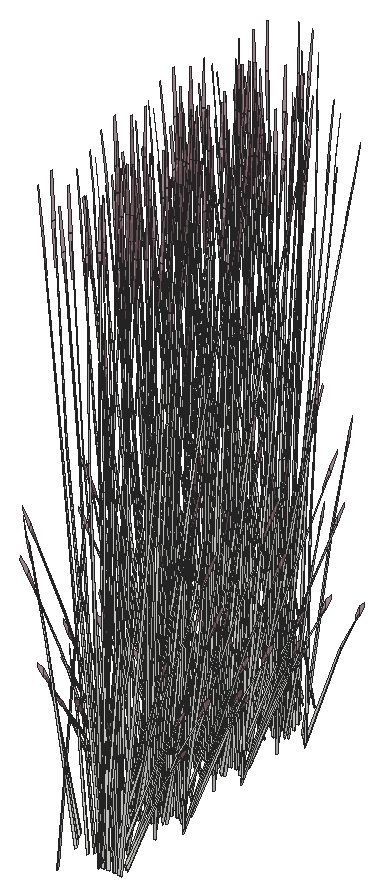
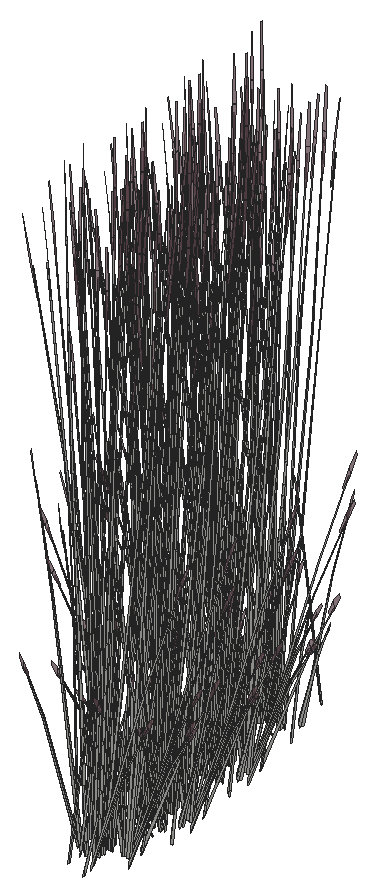
# SketchUp Ruby script. Lengths in inches.
U = 1.inch
M = Sketchup.active_model
def pt(a) = Geom::Point3d.new(a.map { |v| v * U })
def face(e, loops, mat)
  f = e.add_face(loops[0].map { |a| pt(a) })
  loops[1..].each { |l| e.add_face(l.map { |a| pt(a) }).erase! }
  f.material = f.back_material = mat if mat
  f
end
# faces: each face lists its corners as indices into pts; further lists are holes
def faces(e, pts, list, mat = nil) = list.each { |f| face(e, (f[0].is_a?(Array) ? f : [f]).map { |l| l.map { |i| pts[i] } }, mat) }
# xy, xz, yz: faces in a plane at the given z, y or x. An outline is a flat list of corners, or four numbers for a rectangle; further outlines are holes
def ring(l) = l.size == 4 ? [[l[0], l[1]], [l[2], l[1]], [l[2], l[3]], [l[0], l[3]]] : l.each_slice(2).to_a
def flat(e, list, mat, &to3) = list.each { |f| face(e, (f[0].is_a?(Array) ? f : [f]).map { |l| ring(l).map { |u, v| to3.(u, v) } }, mat) }
def xy(e, z, list, mat = nil) = flat(e, list, mat) { |x, y| [x, y, z] }
def xz(e, y, list, mat = nil) = flat(e, list, mat) { |x, z| [x, y, z] }
def yz(e, x, list, mat = nil) = flat(e, list, mat) { |y, z| [x, y, z] }
def lines(e, pts, list) = list.each { |a, b| e.add_line(pt(pts[a]), pt(pts[b])) }
# prism: a flat outline (further loops are holes) pulled along v
def prism(e, loops, v, mat = nil)
  f = face(e, loops, mat); d = Geom::Vector3d.new(v.map { |x| x * U })
  f.pushpull(f.normal.samedirection?(d) ? d.length : -d.length)
end
def box(e, o, s, mat = nil) = prism(e, [[o, [o[0] + s[0], o[1], o[2]], [o[0] + s[0], o[1] + s[1], o[2]], [o[0], o[1] + s[1], o[2]]]], [0, 0, s[2]], mat)
def at(x, y, z, deg = 0) = Geom::Transformation.translation(pt([x, y, z])) * Geom::Transformation.rotation(ORIGIN, Z_AXIS, deg.degrees)
def axes(o, x, y, z) = Geom::Transformation.new([*x, 0, *y, 0, *z, 0, *pt(o).to_a, 1])
def part(name) = M.definitions.add(name)
# library, detail: a bought-in or finely detailed component or shape, given as its bounding box
def library(name, o, s) = part(name).tap { |d| box(d.entities, o, s) }
def detail(e, o, s) = box(e.add_group.entities, o, s)
def put(e, d, t, mat = nil) = e.add_instance(d, t).tap { |i| i.material = mat if mat }
def group(e, t, mat = nil) = e.add_group.tap { |g| g.transformation = t; g.material = mat if mat }.entities
root = M.entities
M.materials.add("LightPink_Translucent").color = [144, 107, 117]
M.materials["LightPink_Translucent"].alpha = 0.75
c1 = part("blade")
p = [[2.15,0.21,22],[0,0.17,0],[0.09,0.45,0],[2.18,0.31,22],[2.29,0.31,22],[0.38,0.45,0],
  [2.48,0.24,33],[2.49,0.24,33],[2.48,0.22,33]]
faces(c1.entities,p,[[0,1,2,3],[4,5,2,3],[6,3,4,7],[8,0,3,6]])
c2 = part("seeds")
p = [[0.3,-0.1,1.38],[-0.01,-0.03,1.59],[-0.01,-0.03,0.03],[0.14,-0.07,-0.07],[0.29,-0.03,3],[0.15,0.01,3.11]]
faces(c2.entities,p,[[0,1,2,3],[1,0,4,5]],"LightPink_Translucent")
c3 = part("blade with seeds")
put(c3.entities,c1,at(0,0,0))
put(c3.entities,c2,axes([2.4,0.25,30.99],[1.5799,-0.05474,1.17369],[-0.12525,1.92788,0.29478],[-0.07173,-0.02425,1.56792]))
put(root,c3,axes([430.54,388.57,152.09],[-0.32198,-0.34356,0.14904],[0.32447,-0.33323,0.29641],[-0.03556,0.07016,1.35512]))
put(root,c3,axes([431.83,388.88,152.34],[-0.2532,0.07787,0.97034],[0.11918,-0.32181,0.71294],[0.13432,0.02202,0.21373]))
put(root,c3,axes([429.12,389.8125,151.86],[-0.41314,-0.21175,0],[0.19883,-0.43999,0],[0,0,1.37455]))
put(root,c3,axes([429.46,389.25,152.08],[-0.40016,-0.37963,-0.21282],[0.33672,-0.42629,0.46574],[-0.10776,0.04441,1.42109]))
put(root,c3,axes([428.41,389.98,152.09],[0.38354,0.23583,0.41945],[-0.22925,0.42288,0],[-0.08735,-0.05371,1.33059]))
put(root,c3,axes([429.76,388.35,152.3],[0.19883,-0.425,0.37796],[0.41314,0.20454,-0.1819],[0,0.09797,1.2135]))
put(root,c3,axes([429.68,388.59,151.9375],[0,0.54548,-0.04762],[-0.51243,0,0],[0,0.01714,1.5153]))
put(root,c3,axes([428.1875,390.22,152],[-0.25622,0.47263,0],[-0.42866,-0.26357,-0.43598],[-0.09763,-0.06003,1.38303]))
put(root,c3,axes([427.72,386.34,152.1875],[0.12932,-0.07441,1.20808],[0.31929,0.22435,-0.25981],[-0.09503,0.19413,0.51652]))
put(root,c3,axes([430.8,388.58,152.09],[0,-0.47166,0.41945],[0.45849,0,0],[0,0.10742,1.33059]))
put(root,c3,axes([429.66,388.93,152.3],[0.44501,-0.02912,0.37796],[0.04024,0.48332,-0.1819],[-0.07967,0.04899,1.2135]))
put(root,c3,axes([429.93,388.44,152.21],[0.38182,-0.13755,0.12232],[0.13371,0.39278,-0.3493],[0,0.08644,1.07074]))
put(root,c3,axes([431.35,389.4,152.1875],[-0.0987,-0.116,1.20808],[0.12841,-0.38374,-0.25981],[0.19968,0.05198,0.51652]))
put(root,c3,axes([429.59,389.82,151.86],[0.41314,0.21175,0],[-0.19883,0.43999,0],[0,0,1.47801]))
put(root,c3,axes([429.75,390.29,151.85],[-0.25302,-0.47428,-0.04344],[0.42866,-0.26357,0.43598],[-0.10563,0.04516,1.38235]))
put(root,c3,axes([429.66,389.14,152.21],[0.30276,0.28338,0.12232],[-0.25254,0.31972,-0.3493],[-0.07029,0.04322,1.07074]))
put(root,c3,axes([429.99,390.02,152.09],[0.38354,-0.23583,0.41945],[0.22925,0.42288,0],[-0.08735,0.05371,1.33059]))
put(root,c3,axes([429.44,389.64,151.9375],[0.17817,0.54185,-0.05079],[-0.50909,0.18987,0],[0.00622,0.01892,1.45452]))
put(root,c3,axes([426.88,389.4,152.1875],[0.14242,0.03872,1.20808],[0.09179,0.39548,-0.25981],[-0.19345,0.07403,0.51652]))
put(root,c3,axes([431.12,388.66,152.01],[0.51243,0,0],[0,0.52715,-0.43598],[0,0.12006,1.38303]))
put(root,c3,axes([430.91,388.93,151.86],[-0.51218,-0.00377,-0.04204],[0,-0.52715,0.42192],[-0.0161,0.12,1.33776]))
put(root,c3,axes([429.8,388.47,152.25],[0.46151,0.22505,-0.2458],[-0.22222,0.475,-0.42242],[0.0145,0.11662,1.34921]))
put(root,c3,axes([426.58,390.22,152.34],[0.17079,-0.21377,0.97034],[0.06739,0.33841,0.71294],[-0.12342,0.0606,0.21373]))
put(root,c3,axes([429.57,389.04,152.25],[0.04775,0.53819,-0.2458],[-0.49736,0.03254,-0.42242],[-0.08758,0.07169,1.34921]))
put(root,c3,axes([428.53,394.79,152.1875],[-0.11649,0.09547,1.20808],[-0.34886,-0.1671,-0.25981],[0.06467,-0.20781,0.51652]))
put(root,c3,axes([426.72,394.61,152.1875],[-0.02482,0.15429,1.20808],[-0.36278,0.12916,-0.25981],[-0.0848,-0.19943,0.51652]))
put(root,c3,axes([427.66,394.27,151.26],[-0.06874,0.01699,1.48974],[-0.38012,-0.19128,-0.22758],[0.00638,-0.15955,0.25375]))
put(root,c3,axes([429.76,390.05,151.97],[0.51304,0.1533,0.25983],[-0.12835,0.54797,-0.30828],[-0.08491,0.06858,1.39295]))
put(root,c3,axes([428.1,394.03,152.34],[0.05257,0.27504,0.97034],[-0.29163,-0.15233,0.71294],[0.03138,-0.14083,0.21373]))
put(root,c3,axes([430.42,390,152.34],[-0.23074,-0.13562,0.97034],[0.29794,-0.1378,0.71294],[0.08036,0.11673,0.21373]))
put(root,c3,axes([430.08,390.34,152],[0.25622,0.47263,0],[-0.42866,0.26357,-0.43598],[-0.09763,0.06003,1.38303]))
put(root,c3,axes([430.48,390.5,151.26],[0.02986,-0.06809,1.48974],[0.37589,-0.20055,-0.22758],[0.11396,0.1038,0.25375]))
put(root,c3,axes([429.86,388.47,152.4],[-0.01119,-0.44408,1.19347],[0.50665,0.11511,0.50532],[-0.11983,0.243,1.12654]))
put(root,c3,axes([427.03,390.44,151.26],[0.05497,0.04712,1.48974],[0.09321,0.43661,-0.22758],[-0.12183,0.0931,0.25375]))
put(root,c3,axes([426.6,394.36,152.34],[0.21377,0.16416,0.97034],[-0.31132,0.09868,0.71294],[-0.06661,-0.12616,0.21373]))
put(root,c3,axes([430.46,390.62,152.25],[-0.26279,-0.01479,0.88755],[0.17355,-0.31417,0.49003],[0.10382,0.11162,0.6962]))
put(root,c3,axes([426.43,394.85,151.26],[-0.0397,0.06213,1.48974],[-0.40116,0.13396,-0.22758],[-0.09691,-0.12186,0.25375]))
put(root,c3,axes([429.34,395.08,151.26],[-0.06134,-0.03716,1.48974],[-0.15755,-0.41512,-0.22758],[0.10629,-0.11265,0.25375]))
put(root,c3,axes([429.6,389.85,152.1875],[0.00723,-0.15635,1.20808],[0.34559,-0.17464,-0.25981],[0.10668,0.18713,0.51652]))
put(root,c3,axes([428.03,391.16,152.34],[-0.01061,-0.28045,0.97034],[0.26501,0.20003,0.71294],[-0.05212,0.13367,0.21373]))
put(root,c3,axes([427.03,395.17,152],[-0.25622,-0.47263,0],[0.42866,-0.26357,-0.43598],[0.09763,-0.06003,1.38303]))
put(root,c3,axes([428.73,390.49,151.26],[0.06632,-0.02567,1.48974],[0.39894,0.14126,-0.22758],[0.01167,0.15921,0.25375]))
put(root,c3,axes([427.59,394.6,151.8],[-0.28319,0.27058,-0.03288],[-0.25948,-0.29635,-0.1491],[-0.01827,-0.08397,0.4918]))
put(root,c3,axes([427.8125,390.55,152.38],[0.37228,-0.08352,0.05498],[0.08559,0.3365,-0.7291],[-0.0236,0.17034,0.65354]))
put(root,c3,axes([429.65,395.91,152.1875],[-0.1464,-0.01397,1.20808],[-0.14998,-0.37477,-0.25981],[0.17985,-0.10602,0.51652]))
put(root,c3,axes([429.82,395.22,152.34],[-0.1365,0.2401,0.97034],[-0.11733,-0.32258,0.71294],[0.11274,-0.08083,0.21373]))
put(root,c3,axes([427.72,390.91,152.1875],[0.12932,-0.07441,1.20808],[0.31929,0.22435,-0.25981],[-0.09503,0.19413,0.51652]))
put(root,c3,axes([427.53,396.47,152.25],[-0.04775,-0.53819,-0.2458],[0.49736,-0.03254,-0.42242],[0.08758,-0.07169,1.34921]))
put(root,c3,axes([426.18,395.09,151.8],[-0.11822,0.38513,-0.03288],[-0.36385,-0.11847,-0.1491],[-0.05524,-0.06299,0.4918]))
put(root,c3,axes([427.3,397.04,152.25],[-0.46151,-0.22505,-0.2458],[0.22222,-0.475,-0.42242],[-0.0145,-0.11662,1.34921]))
put(root,c3,axes([425.99,396.85,152],[-0.51243,0,0],[0,-0.52715,-0.43598],[0,-0.12006,1.38303]))
put(root,c3,axes([426.07,395.91,152.1875],[0.08001,0.13132,1.20808],[-0.18437,0.35694,-0.25981],[-0.18931,-0.08532,0.51652]))
put(root,c3,axes([426.38,396.71,151.97],[-0.38118,0.39654,0.25983],[-0.38142,-0.39237,-0.30828],[-0.01331,-0.11261,1.39295]))
put(root,c3,axes([427.59,396.9,152.06],[0.46174,0.2286,0.2033],[-0.22222,0.475,0.42242],[0,-0.1095,1.35626]))
put(root,c3,axes([427.41,397.54,152.06],[0.10862,-0.55889,-0.19793],[0.515,0.09742,0.43313],[-0.08999,-0.07718,1.32161]))
put(root,c3,axes([425.6,396.3,152.34],[0.26163,-0.03375,0.97034],[-0.16596,0.29737,0.71294],[-0.12929,-0.04461,0.21373]))
put(root,c3,axes([427.45,396.58,152.3],[-0.44501,0.02912,0.37796],[-0.04024,-0.48332,-0.1819],[0.07967,-0.04899,1.2135]))
put(root,c3,axes([426.3,396.93,152.09],[0,0.47166,0.41945],[-0.45849,0,0],[0,-0.10742,1.33059]))
put(root,c3,axes([428.91,395.29,152.01],[0.25622,-0.47263,0],[0.42866,0.26357,-0.43598],[0.09763,0.06003,1.38303]))
put(root,c3,axes([427.43,396.75,151.99],[0.17817,0.52741,0.38653],[-0.50909,0.1834,0.15168],[0.00622,-0.09691,1.34202]))
put(root,c3,axes([429.92,397.16,151.67],[-0.26394,0.0566,1.1961],[-0.04201,-0.45055,0.06846],[0.18486,-0.06819,0.68062]))
put(root,c3,axes([430.4,396.76,151.91],[-0.25407,-0.3016,-0.05481],[0.27826,-0.27635,-0.2485],[0.07884,-0.01946,0.81966]))
put(root,c3,axes([427.34,397.17,152.3],[-0.19883,0.425,0.37796],[-0.41314,-0.20454,-0.1819],[0,-0.09797,1.2135]))
put(root,c3,axes([428.07,396.8,151.86],[0,-0.54574,0],[0.51243,0,0],[0,0,1.51605]))
put(root,c3,axes([428.69,395.53,152.09],[-0.38354,-0.23583,0.41945],[0.22925,-0.42288,0],[0.08735,0.05371,1.33059]))
put(root,c3,axes([427.83,396.45,151.99],[-0.33979,0.42804,0.38653],[-0.40368,-0.37784,0.15168],[0.08192,-0.04272,1.34202]))
put(root,c3,axes([428.2,397.22,151.94],[-0.38118,-0.40596,-0.0518],[0.38142,-0.40621,0],[-0.01331,-0.01418,1.48322]))
put(root,c3,axes([427.24,395.75,152.09],[-0.11838,0.46875,0.14904],[-0.43321,-0.13265,0.29641],[0.07483,-0.00228,1.35512]))
put(root,c3,axes([427.06,396.125,151.35],[-0.40337,0.18883,1.08919],[-0.12839,-0.54182,0.42321],[0.24769,0.00901,1.23883]))
put(root,c3,axes([428.14,396.27,152.21],[0.07906,-0.42093,0.12232],[0.38625,0.07307,-0.3493],[0.07029,0.04322,1.07074]))
put(root,c3,axes([427.47,397.27,151.99],[0.51796,0.09937,0.38653],[-0.10541,0.56124,0.15168],[-0.07569,-0.05419,1.34202]))
put(root,c3,axes([430.21,396.86,151.26],[-0.02142,-0.07161,1.48974],[0.14855,-0.41887,-0.22758],[0.14984,-0.00603,0.25375]))
put(root,c3,axes([425.79,396.79,151.26],[0.01039,0.07433,1.48974],[-0.20952,0.38819,-0.22758],[-0.14882,-0.01957,0.25375]))
put(root,c3,axes([427.98,396.38,152.3],[-0.24618,-0.39589,0.37796],[0.37289,-0.27878,-0.1819],[0.07967,0.04899,1.2135]))
put(root,c3,axes([427.2,398.16,152.09],[0.44036,-0.12519,0.14904],[0.10874,0.46588,0.29641],[-0.03927,-0.06788,1.35512]))
put(root,c3,axes([428.1,396.4,152.25],[0.41376,-0.31314,-0.2458],[0.27514,0.44246,-0.42242],[0.10209,0.04493,1.34921]))
put(root,c3,axes([428.42,396.92,151.86],[0.45849,0,0],[0,0.4883,0],[0,0,1.50718]))
put(root,c3,axes([427.64,397.53,152.25],[-0.41376,0.31314,-0.2458],[-0.27514,-0.44246,-0.42242],[-0.10209,-0.04493,1.34921]))
put(root,c3,axes([428.55,395.77,152.09],[-0.44036,0.12519,0.14904],[-0.10874,-0.46588,0.29641],[0.03927,0.06788,1.35512]))
put(root,c3,axes([428.27,396.67,152.01],[-0.51796,-0.09937,0.41563],[0.10541,-0.56124,0.1631],[0.07569,0.05419,1.44303]))
put(root,c3,axes([427.86,398.05,151.86],[-0.13371,-0.40664,0],[0.38182,-0.1424,0],[0,0,1.30413]))
put(root,c3,axes([427.6,397.67,152.21],[-0.07906,0.42093,0.12232],[-0.38625,-0.07307,-0.3493],[-0.07029,-0.04322,1.07074]))
put(root,c3,axes([428.36,398,151.85],[0.43024,-0.16003,-0.16218],[0.15118,0.46099,0.00007],[0.04749,-0.01769,1.46908]))
put(root,c3,axes([428.51,398.19,152.09],[0.11838,-0.46875,0.14904],[0.43321,0.13265,0.29641],[-0.07483,0.00228,1.35512]))
put(root,c3,axes([428.41,397.125,151.87],[0.28606,0.30466,0],[-0.28606,0.30466,0],[0,0,1.42996]))
put(root,c3,axes([429.18,396.99,152.09],[-0.32198,-0.34356,0.14904],[0.32447,-0.33323,0.29641],[-0.03556,0.07016,1.35512]))
put(root,c3,axes([430.47,397.31,152.34],[-0.2532,0.07787,0.97034],[0.11918,-0.32181,0.71294],[0.13432,0.02202,0.21373]))
put(root,c3,axes([427.76,398.24,151.86],[-0.41314,-0.21175,0],[0.19883,-0.43999,0],[0,0,1.37455]))
put(root,c3,axes([428.11,397.67,152.08],[-0.40016,-0.37963,-0.21282],[0.33672,-0.42629,0.46574],[-0.10776,0.04441,1.42109]))
put(root,c3,axes([427.05,398.4,152.09],[0.38354,0.23583,0.41945],[-0.22925,0.42288,0],[-0.08735,-0.05371,1.33059]))
put(root,c3,axes([428.4,396.77,152.3],[0.19883,-0.425,0.37796],[0.41314,0.20454,-0.1819],[0,0.09797,1.2135]))
put(root,c3,axes([428.33,397.01,151.9375],[0,0.54548,-0.04762],[-0.51243,0,0],[0,0.01714,1.5153]))
put(root,c3,axes([426.83,398.65,152],[-0.25622,0.47263,0],[-0.42866,-0.26357,-0.43598],[-0.09763,-0.06003,1.38303]))
put(root,c3,axes([429.45,397.01,152.09],[0,-0.47166,0.41945],[0.45849,0,0],[0,0.10742,1.33059]))
put(root,c3,axes([428.3,397.36,152.3],[0.44501,-0.02912,0.37796],[0.04024,0.48332,-0.1819],[-0.07967,0.04899,1.2135]))
put(root,c3,axes([428.58,396.87,152.21],[0.38182,-0.13755,0.12232],[0.13371,0.39278,-0.3493],[0,0.08644,1.07074]))
put(root,c3,axes([430,397.82,152.1875],[-0.0987,-0.116,1.20808],[0.12841,-0.38374,-0.25981],[0.19968,0.05198,0.51652]))
put(root,c3,axes([428.23,398.25,151.86],[0.41314,0.21175,0],[-0.19883,0.43999,0],[0,0,1.47801]))
put(root,c3,axes([427.44,402.36,152.1875],[-0.11649,0.09547,1.20808],[-0.34886,-0.1671,-0.25981],[0.06467,-0.20781,0.51652]))
put(root,c3,axes([428.4,398.71,151.85],[-0.25302,-0.47428,-0.04344],[0.42866,-0.26357,0.43598],[-0.10563,0.04516,1.38235]))
put(root,c3,axes([425.64,402.18,152.1875],[-0.02482,0.15429,1.20808],[-0.36278,0.12916,-0.25981],[-0.0848,-0.19943,0.51652]))
put(root,c3,axes([428.31,397.57,152.21],[0.30276,0.28338,0.12232],[-0.25254,0.31972,-0.3493],[-0.07029,0.04322,1.07074]))
put(root,c3,axes([426.57,401.85,151.26],[-0.06874,0.01699,1.48974],[-0.38012,-0.19128,-0.22758],[0.00638,-0.15955,0.25375]))
put(root,c3,axes([428.63,398.44,152.09],[0.38354,-0.23583,0.41945],[0.22925,0.42288,0],[-0.08735,0.05371,1.33059]))
put(root,c3,axes([428.08,398.07,151.9375],[0.17817,0.54185,-0.05079],[-0.50909,0.18987,0],[0.00622,0.01892,1.45452]))
put(root,c3,axes([425.52,397.82,152.1875],[0.14242,0.03872,1.20808],[0.09179,0.39548,-0.25981],[-0.19345,0.07403,0.51652]))
put(root,c3,axes([429.76,397.09,152.01],[0.51243,0,0],[0,0.52715,-0.43598],[0,0.12006,1.38303]))
put(root,c3,axes([429.55,397.36,151.86],[-0.51218,-0.00377,-0.04204],[0,-0.52715,0.42192],[-0.0161,0.12,1.33776]))
put(root,c3,axes([427.01,401.6,152.34],[0.05257,0.27504,0.97034],[-0.29163,-0.15233,0.71294],[0.03138,-0.14083,0.21373]))
put(root,c3,axes([428.45,396.9,152.25],[0.46151,0.22505,-0.2458],[-0.22222,0.475,-0.42242],[0.0145,0.11662,1.34921]))
put(root,c3,axes([425.23,398.65,152.34],[0.17079,-0.21377,0.97034],[0.06739,0.33841,0.71294],[-0.12342,0.0606,0.21373]))
put(root,c3,axes([428.22,397.46,152.25],[0.04775,0.53819,-0.2458],[-0.49736,0.03254,-0.42242],[-0.08758,0.07169,1.34921]))
put(root,c3,axes([425.51,401.94,152.34],[0.21377,0.16416,0.97034],[-0.31132,0.09868,0.71294],[-0.06661,-0.12616,0.21373]))
put(root,c3,axes([428.41,398.47,151.97],[0.51304,0.1533,0.25983],[-0.12835,0.54797,-0.30828],[-0.08491,0.06858,1.39295]))
put(root,c3,axes([429.0625,398.42,152.34],[-0.23074,-0.13562,0.97034],[0.29794,-0.1378,0.71294],[0.08036,0.11673,0.21373]))
put(root,c3,axes([425.35,402.43,151.26],[-0.0397,0.06213,1.48974],[-0.40116,0.13396,-0.22758],[-0.09691,-0.12186,0.25375]))
put(root,c3,axes([428.26,402.66,151.26],[-0.06134,-0.03716,1.48974],[-0.15755,-0.41512,-0.22758],[0.10629,-0.11265,0.25375]))
put(root,c3,axes([428.72,398.77,152],[0.25622,0.47263,0],[-0.42866,0.26357,-0.43598],[-0.09763,0.06003,1.38303]))
put(root,c3,axes([429.13,398.93,151.26],[0.02986,-0.06809,1.48974],[0.37589,-0.20055,-0.22758],[0.11396,0.1038,0.25375]))
put(root,c3,axes([428.5,396.9,152.4],[-0.01119,-0.44408,1.19347],[0.50665,0.11511,0.50532],[-0.11983,0.243,1.12654]))
put(root,c3,axes([425.68,398.87,151.26],[0.05497,0.04712,1.48974],[0.09321,0.43661,-0.22758],[-0.12183,0.0931,0.25375]))
put(root,c3,axes([425.94,402.75,152],[-0.25622,-0.47263,0],[0.42866,-0.26357,-0.43598],[0.09763,-0.06003,1.38303]))
put(root,c3,axes([429.1,399.04,152.25],[-0.26279,-0.01479,0.88755],[0.17355,-0.31417,0.49003],[0.10382,0.11162,0.6962]))
put(root,c3,axes([426.5,402.18,151.8],[-0.28319,0.27058,-0.03288],[-0.25948,-0.29635,-0.1491],[-0.01827,-0.08397,0.4918]))
put(root,c3,axes([428.24,398.28,152.1875],[0.00723,-0.15635,1.20808],[0.34559,-0.17464,-0.25981],[0.10668,0.18713,0.51652]))
put(root,c3,axes([428.57,403.49,152.1875],[-0.1464,-0.01397,1.20808],[-0.14998,-0.37477,-0.25981],[0.17985,-0.10602,0.51652]))
put(root,c3,axes([428.73,402.8,152.34],[-0.1365,0.2401,0.97034],[-0.11733,-0.32258,0.71294],[0.11274,-0.08083,0.21373]))
put(root,c3,axes([426.67,399.58,152.34],[-0.01061,-0.28045,0.97034],[0.26501,0.20003,0.71294],[-0.05212,0.13367,0.21373]))
put(root,c3,axes([427.37,398.91,151.26],[0.06632,-0.02567,1.48974],[0.39894,0.14126,-0.22758],[0.01167,0.15921,0.25375]))
put(root,c3,axes([426.44,404.05,152.25],[-0.04775,-0.53819,-0.2458],[0.49736,-0.03254,-0.42242],[0.08758,-0.07169,1.34921]))
put(root,c3,axes([426.45,398.98,152.38],[0.37228,-0.08352,0.05498],[0.08559,0.3365,-0.7291],[-0.0236,0.17034,0.65354]))
put(root,c3,axes([425.1,402.67,151.8],[-0.11822,0.38513,-0.03288],[-0.36385,-0.11847,-0.1491],[-0.05524,-0.06299,0.4918]))
put(root,c3,axes([426.21,404.62,152.25],[-0.46151,-0.22505,-0.2458],[0.22222,-0.475,-0.42242],[-0.0145,-0.11662,1.34921]))
put(root,c3,axes([424.9,404.43,152],[-0.51243,0,0],[0,-0.52715,-0.43598],[0,-0.12006,1.38303]))
put(root,c3,axes([424.99,403.49,152.1875],[0.08001,0.13132,1.20808],[-0.18437,0.35694,-0.25981],[-0.18931,-0.08532,0.51652]))
put(root,c3,axes([425.3,404.29,151.97],[-0.38118,0.39654,0.25983],[-0.38142,-0.39237,-0.30828],[-0.01331,-0.11261,1.39295]))
put(root,c3,axes([426.36,399.33,152.1875],[0.12932,-0.07441,1.20808],[0.31929,0.22435,-0.25981],[-0.09503,0.19413,0.51652]))
put(root,c3,axes([426.51,404.47,152.06],[0.46174,0.2286,0.2033],[-0.22222,0.475,0.42242],[0,-0.1095,1.35626]))
put(root,c3,axes([426.33,405.12,152.06],[0.10862,-0.55889,-0.19793],[0.515,0.09742,0.43313],[-0.08999,-0.07718,1.32161]))
put(root,c3,axes([424.51,403.88,152.34],[0.26163,-0.03375,0.97034],[-0.16596,0.29737,0.71294],[-0.12929,-0.04461,0.21373]))
put(root,c3,axes([426.36,404.15,152.3],[-0.44501,0.02912,0.37796],[-0.04024,-0.48332,-0.1819],[0.07967,-0.04899,1.2135]))
put(root,c3,axes([425.21,404.51,152.09],[0,0.47166,0.41945],[-0.45849,0,0],[0,-0.10742,1.33059]))
put(root,c3,axes([427.83,402.87,152.01],[0.25622,-0.47263,0],[0.42866,0.26357,-0.43598],[0.09763,0.06003,1.38303]))
put(root,c3,axes([426.35,404.33,151.99],[0.17817,0.52741,0.38653],[-0.50909,0.1834,0.15168],[0.00622,-0.09691,1.34202]))
put(root,c3,axes([428.84,404.73,151.67],[-0.26394,0.0566,1.1961],[-0.04201,-0.45055,0.06846],[0.18486,-0.06819,0.68062]))
put(root,c3,axes([429.32,404.33,151.91],[-0.25407,-0.3016,-0.05481],[0.27826,-0.27635,-0.2485],[0.07884,-0.01946,0.81966]))
put(root,c3,axes([426.26,404.74,152.3],[-0.19883,0.425,0.37796],[-0.41314,-0.20454,-0.1819],[0,-0.09797,1.2135]))
put(root,c3,axes([426.99,404.375,151.86],[0,-0.54574,0],[0.51243,0,0],[0,0,1.51605]))
put(root,c3,axes([427.61,403.11,152.09],[-0.38354,-0.23583,0.41945],[0.22925,-0.42288,0],[0.08735,0.05371,1.33059]))
put(root,c3,axes([426.74,404.03,151.99],[-0.33979,0.42804,0.38653],[-0.40368,-0.37784,0.15168],[0.08192,-0.04272,1.34202]))
put(root,c3,axes([427.11,404.8,151.94],[-0.38118,-0.40596,-0.0518],[0.38142,-0.40621,0],[-0.01331,-0.01418,1.48322]))
put(root,c3,axes([426.15,403.32,152.09],[-0.11838,0.46875,0.14904],[-0.43321,-0.13265,0.29641],[0.07483,-0.00228,1.35512]))
put(root,c3,axes([425.97,403.7,151.35],[-0.40337,0.18883,1.08919],[-0.12839,-0.54182,0.42321],[0.24769,0.00901,1.23883]))
put(root,c3,axes([427.06,403.85,152.21],[0.07906,-0.42093,0.12232],[0.38625,0.07307,-0.3493],[0.07029,0.04322,1.07074]))
put(root,c3,axes([426.39,404.85,151.99],[0.51796,0.09937,0.38653],[-0.10541,0.56124,0.15168],[-0.07569,-0.05419,1.34202]))
put(root,c3,axes([429.125,404.4375,151.26],[-0.02142,-0.07161,1.48974],[0.14855,-0.41887,-0.22758],[0.14984,-0.00603,0.25375]))
put(root,c3,axes([424.7,404.37,151.26],[0.01039,0.07433,1.48974],[-0.20952,0.38819,-0.22758],[-0.14882,-0.01957,0.25375]))
put(root,c3,axes([426.89,403.96,152.3],[-0.24618,-0.39589,0.37796],[0.37289,-0.27878,-0.1819],[0.07967,0.04899,1.2135]))
put(root,c3,axes([426.11,405.74,152.09],[0.44036,-0.12519,0.14904],[0.10874,0.46588,0.29641],[-0.03927,-0.06788,1.35512]))
put(root,c3,axes([427.02,403.98,152.25],[0.41376,-0.31314,-0.2458],[0.27514,0.44246,-0.42242],[0.10209,0.04493,1.34921]))
put(root,c3,axes([427.33,404.5,151.86],[0.45849,0,0],[0,0.4883,0],[0,0,1.50718]))
put(root,c3,axes([426.56,405.11,152.25],[-0.41376,0.31314,-0.2458],[-0.27514,-0.44246,-0.42242],[-0.10209,-0.04493,1.34921]))
put(root,c3,axes([427.46,403.35,152.09],[-0.44036,0.12519,0.14904],[-0.10874,-0.46588,0.29641],[0.03927,0.06788,1.35512]))
put(root,c3,axes([427.1875,404.25,152.01],[-0.51796,-0.09937,0.41563],[0.10541,-0.56124,0.1631],[0.07569,0.05419,1.44303]))
put(root,c3,axes([426.77,405.63,151.86],[-0.13371,-0.40664,0],[0.38182,-0.1424,0],[0,0,1.30413]))
put(root,c3,axes([426.52,405.25,152.21],[-0.07906,0.42093,0.12232],[-0.38625,-0.07307,-0.3493],[-0.07029,-0.04322,1.07074]))
put(root,c3,axes([427.27,405.58,151.85],[0.43024,-0.16003,-0.16218],[0.15118,0.46099,0.00007],[0.04749,-0.01769,1.46908]))
put(root,c3,axes([427.42,405.77,152.09],[0.11838,-0.46875,0.14904],[0.43321,0.13265,0.29641],[-0.07483,0.00228,1.35512]))
put(root,c3,axes([427.32,404.71,151.87],[0.28606,0.30466,0],[-0.28606,0.30466,0],[0,0,1.42996]))
put(root,c3,axes([427.59,408.91,152.1875],[-0.11649,0.09547,1.20808],[-0.34886,-0.1671,-0.25981],[0.06467,-0.20781,0.51652]))
put(root,c3,axes([428.1,404.57,152.09],[-0.32198,-0.34356,0.14904],[0.32447,-0.33323,0.29641],[-0.03556,0.07016,1.35512]))
put(root,c3,axes([429.39,404.89,152.34],[-0.2532,0.07787,0.97034],[0.11918,-0.32181,0.71294],[0.13432,0.02202,0.21373]))
put(root,c3,axes([425.78,408.73,152.1875],[-0.02482,0.15429,1.20808],[-0.36278,0.12916,-0.25981],[-0.0848,-0.19943,0.51652]))
put(root,c3,axes([426.68,405.82,151.86],[-0.41314,-0.21175,0],[0.19883,-0.43999,0],[0,0,1.37455]))
put(root,c3,axes([427.02,405.25,152.08],[-0.40016,-0.37963,-0.21282],[0.33672,-0.42629,0.46574],[-0.10776,0.04441,1.42109]))
put(root,c3,axes([425.97,405.98,152.09],[0.38354,0.23583,0.41945],[-0.22925,0.42288,0],[-0.08735,-0.05371,1.33059]))
put(root,c3,axes([426.72,408.39,151.26],[-0.06874,0.01699,1.48974],[-0.38012,-0.19128,-0.22758],[0.00638,-0.15955,0.25375]))
put(root,c3,axes([427.32,404.35,152.3],[0.19883,-0.425,0.37796],[0.41314,0.20454,-0.1819],[0,0.09797,1.2135]))
put(root,c3,axes([427.24,404.59,151.9375],[0,0.54548,-0.04762],[-0.51243,0,0],[0,0.01714,1.5153]))
put(root,c3,axes([425.75,406.23,152],[-0.25622,0.47263,0],[-0.42866,-0.26357,-0.43598],[-0.09763,-0.06003,1.38303]))
put(root,c3,axes([428.36,404.59,152.09],[0,-0.47166,0.41945],[0.45849,0,0],[0,0.10742,1.33059]))
put(root,c3,axes([427.21,404.9375,152.3],[0.44501,-0.02912,0.37796],[0.04024,0.48332,-0.1819],[-0.07967,0.04899,1.2135]))
put(root,c3,axes([427.49,404.45,152.21],[0.38182,-0.13755,0.12232],[0.13371,0.39278,-0.3493],[0,0.08644,1.07074]))
put(root,c3,axes([427.16,408.15,152.34],[0.05257,0.27504,0.97034],[-0.29163,-0.15233,0.71294],[0.03138,-0.14083,0.21373]))
put(root,c3,axes([428.91,405.4,152.1875],[-0.0987,-0.116,1.20808],[0.12841,-0.38374,-0.25981],[0.19968,0.05198,0.51652]))
put(root,c3,axes([427.15,405.82,151.86],[0.41314,0.21175,0],[-0.19883,0.43999,0],[0,0,1.47801]))
put(root,c3,axes([427.3125,406.29,151.85],[-0.25302,-0.47428,-0.04344],[0.42866,-0.26357,0.43598],[-0.10563,0.04516,1.38235]))
put(root,c3,axes([427.22,405.15,152.21],[0.30276,0.28338,0.12232],[-0.25254,0.31972,-0.3493],[-0.07029,0.04322,1.07074]))
put(root,c3,axes([425.66,408.48,152.34],[0.21377,0.16416,0.97034],[-0.31132,0.09868,0.71294],[-0.06661,-0.12616,0.21373]))
put(root,c3,axes([427.54,406.02,152.09],[0.38354,-0.23583,0.41945],[0.22925,0.42288,0],[-0.08735,0.05371,1.33059]))
put(root,c3,axes([427,405.65,151.9375],[0.17817,0.54185,-0.05079],[-0.50909,0.18987,0],[0.00622,0.01892,1.45452]))
put(root,c3,axes([424.4375,405.4,152.1875],[0.14242,0.03872,1.20808],[0.09179,0.39548,-0.25981],[-0.19345,0.07403,0.51652]))
put(root,c3,axes([425.49,408.98,151.26],[-0.0397,0.06213,1.48974],[-0.40116,0.13396,-0.22758],[-0.09691,-0.12186,0.25375]))
put(root,c3,axes([428.67,404.67,152.01],[0.51243,0,0],[0,0.52715,-0.43598],[0,0.12006,1.38303]))
put(root,c3,axes([428.47,404.9375,151.86],[-0.51218,-0.00377,-0.04204],[0,-0.52715,0.42192],[-0.0161,0.12,1.33776]))
put(root,c3,axes([427.36,404.48,152.25],[0.46151,0.22505,-0.2458],[-0.22222,0.475,-0.42242],[0.0145,0.11662,1.34921]))
put(root,c3,axes([428.4,409.21,151.26],[-0.06134,-0.03716,1.48974],[-0.15755,-0.41512,-0.22758],[0.10629,-0.11265,0.25375]))
put(root,c3,axes([424.14,406.23,152.34],[0.17079,-0.21377,0.97034],[0.06739,0.33841,0.71294],[-0.12342,0.0606,0.21373]))
put(root,c3,axes([427.13,405.04,152.25],[0.04775,0.53819,-0.2458],[-0.49736,0.03254,-0.42242],[-0.08758,0.07169,1.34921]))
put(root,c3,axes([426.09,409.3,152],[-0.25622,-0.47263,0],[0.42866,-0.26357,-0.43598],[0.09763,-0.06003,1.38303]))
put(root,c3,axes([426.65,408.73,151.8],[-0.28319,0.27058,-0.03288],[-0.25948,-0.29635,-0.1491],[-0.01827,-0.08397,0.4918]))
put(root,c3,axes([427.32,406.05,151.97],[0.51304,0.1533,0.25983],[-0.12835,0.54797,-0.30828],[-0.08491,0.06858,1.39295]))
put(root,c3,axes([427.98,406,152.34],[-0.23074,-0.13562,0.97034],[0.29794,-0.1378,0.71294],[0.08036,0.11673,0.21373]))
put(root,c3,axes([428.71,410.04,152.1875],[-0.1464,-0.01397,1.20808],[-0.14998,-0.37477,-0.25981],[0.17985,-0.10602,0.51652]))
put(root,c3,axes([428.88,409.35,152.34],[-0.1365,0.2401,0.97034],[-0.11733,-0.32258,0.71294],[0.11274,-0.08083,0.21373]))
put(root,c3,axes([427.63,406.35,152],[0.25622,0.47263,0],[-0.42866,0.26357,-0.43598],[-0.09763,0.06003,1.38303]))
put(root,c3,axes([428.04,406.51,151.26],[0.02986,-0.06809,1.48974],[0.37589,-0.20055,-0.22758],[0.11396,0.1038,0.25375]))
put(root,c3,axes([427.42,404.48,152.4],[-0.01119,-0.44408,1.19347],[0.50665,0.11511,0.50532],[-0.11983,0.243,1.12654]))
put(root,c3,axes([424.59,406.45,151.26],[0.05497,0.04712,1.48974],[0.09321,0.43661,-0.22758],[-0.12183,0.0931,0.25375]))
put(root,c3,axes([426.59,410.6,152.25],[-0.04775,-0.53819,-0.2458],[0.49736,-0.03254,-0.42242],[0.08758,-0.07169,1.34921]))
put(root,c3,axes([428.01,406.62,152.25],[-0.26279,-0.01479,0.88755],[0.17355,-0.31417,0.49003],[0.10382,0.11162,0.6962]))
put(root,c3,axes([425.24,409.22,151.8],[-0.11822,0.38513,-0.03288],[-0.36385,-0.11847,-0.1491],[-0.05524,-0.06299,0.4918]))
put(root,c3,axes([426.36,411.16,152.25],[-0.46151,-0.22505,-0.2458],[0.22222,-0.475,-0.42242],[-0.0145,-0.11662,1.34921]))
put(root,c3,axes([425.05,410.98,152],[-0.51243,0,0],[0,-0.52715,-0.43598],[0,-0.12006,1.38303]))
put(root,c3,axes([425.13,410.03,152.1875],[0.08001,0.13132,1.20808],[-0.18437,0.35694,-0.25981],[-0.18931,-0.08532,0.51652]))
put(root,c3,axes([427.16,405.86,152.1875],[0.00723,-0.15635,1.20808],[0.34559,-0.17464,-0.25981],[0.10668,0.18713,0.51652]))
put(root,c3,axes([425.59,407.16,152.34],[-0.01061,-0.28045,0.97034],[0.26501,0.20003,0.71294],[-0.05212,0.13367,0.21373]))
put(root,c3,axes([425.44,410.84,151.97],[-0.38118,0.39654,0.25983],[-0.38142,-0.39237,-0.30828],[-0.01331,-0.11261,1.39295]))
put(root,c3,axes([426.29,406.49,151.26],[0.06632,-0.02567,1.48974],[0.39894,0.14126,-0.22758],[0.01167,0.15921,0.25375]))
put(root,c3,axes([426.65,411.02,152.06],[0.46174,0.2286,0.2033],[-0.22222,0.475,0.42242],[0,-0.1095,1.35626]))
put(root,c3,axes([426.47,411.66,152.06],[0.10862,-0.55889,-0.19793],[0.515,0.09742,0.43313],[-0.08999,-0.07718,1.32161]))
put(root,c3,axes([425.37,406.55,152.38],[0.37228,-0.08352,0.05498],[0.08559,0.3365,-0.7291],[-0.0236,0.17034,0.65354]))
put(root,c3,axes([424.66,410.43,152.34],[0.26163,-0.03375,0.97034],[-0.16596,0.29737,0.71294],[-0.12929,-0.04461,0.21373]))
put(root,c3,axes([426.51,410.7,152.3],[-0.44501,0.02912,0.37796],[-0.04024,-0.48332,-0.1819],[0.07967,-0.04899,1.2135]))
put(root,c3,axes([425.36,411.06,152.09],[0,0.47166,0.41945],[-0.45849,0,0],[0,-0.10742,1.33059]))
put(root,c3,axes([427.97,409.41,152.01],[0.25622,-0.47263,0],[0.42866,0.26357,-0.43598],[0.09763,0.06003,1.38303]))
put(root,c3,axes([426.49,410.88,151.99],[0.17817,0.52741,0.38653],[-0.50909,0.1834,0.15168],[0.00622,-0.09691,1.34202]))
put(root,c3,axes([428.98,411.28,151.67],[-0.26394,0.0566,1.1961],[-0.04201,-0.45055,0.06846],[0.18486,-0.06819,0.68062]))
put(root,c3,axes([429.46,410.88,151.91],[-0.25407,-0.3016,-0.05481],[0.27826,-0.27635,-0.2485],[0.07884,-0.01946,0.81966]))
put(root,c3,axes([426.4,411.29,152.3],[-0.19883,0.425,0.37796],[-0.41314,-0.20454,-0.1819],[0,-0.09797,1.2135]))
put(root,c3,axes([427.13,410.92,151.86],[0,-0.54574,0],[0.51243,0,0],[0,0,1.51605]))
put(root,c3,axes([427.75,409.66,152.09],[-0.38354,-0.23583,0.41945],[0.22925,-0.42288,0],[0.08735,0.05371,1.33059]))
put(root,c3,axes([426.89,410.58,151.99],[-0.33979,0.42804,0.38653],[-0.40368,-0.37784,0.15168],[0.08192,-0.04272,1.34202]))
put(root,c3,axes([425.28,406.91,152.1875],[0.12932,-0.07441,1.20808],[0.31929,0.22435,-0.25981],[-0.09503,0.19413,0.51652]))
put(root,c3,axes([427.26,411.35,151.94],[-0.38118,-0.40596,-0.0518],[0.38142,-0.40621,0],[-0.01331,-0.01418,1.48322]))
put(root,c3,axes([426.3,409.875,152.09],[-0.11838,0.46875,0.14904],[-0.43321,-0.13265,0.29641],[0.07483,-0.00228,1.35512]))
put(root,c3,axes([426.12,410.25,151.35],[-0.40337,0.18883,1.08919],[-0.12839,-0.54182,0.42321],[0.24769,0.00901,1.23883]))
put(root,c3,axes([427.2,410.39,152.21],[0.07906,-0.42093,0.12232],[0.38625,0.07307,-0.3493],[0.07029,0.04322,1.07074]))
put(root,c3,axes([427.52,414.3,152.1875],[-0.11649,0.09547,1.20808],[-0.34886,-0.1671,-0.25981],[0.06467,-0.20781,0.51652]))
put(root,c3,axes([426.53,411.39,151.99],[0.51796,0.09937,0.38653],[-0.10541,0.56124,0.15168],[-0.07569,-0.05419,1.34202]))
put(root,c3,axes([429.27,410.99,151.26],[-0.02142,-0.07161,1.48974],[0.14855,-0.41887,-0.22758],[0.14984,-0.00603,0.25375]))
put(root,c3,axes([424.85,410.91,151.26],[0.01039,0.07433,1.48974],[-0.20952,0.38819,-0.22758],[-0.14882,-0.01957,0.25375]))
put(root,c3,axes([425.71,414.11,152.1875],[-0.02482,0.15429,1.20808],[-0.36278,0.12916,-0.25981],[-0.0848,-0.19943,0.51652]))
put(root,c3,axes([427.04,410.51,152.3],[-0.24618,-0.39589,0.37796],[0.37289,-0.27878,-0.1819],[0.07967,0.04899,1.2135]))
put(root,c3,axes([426.65,413.78,151.26],[-0.06874,0.01699,1.48974],[-0.38012,-0.19128,-0.22758],[0.00638,-0.15955,0.25375]))
put(root,c3,axes([426.26,412.29,152.09],[0.44036,-0.12519,0.14904],[0.10874,0.46588,0.29641],[-0.03927,-0.06788,1.35512]))
put(root,c3,axes([427.16,410.53,152.25],[0.41376,-0.31314,-0.2458],[0.27514,0.44246,-0.42242],[0.10209,0.04493,1.34921]))
put(root,c3,axes([427.48,411.04,151.86],[0.45849,0,0],[0,0.4883,0],[0,0,1.50718]))
put(root,c3,axes([426.7,411.66,152.25],[-0.41376,0.31314,-0.2458],[-0.27514,-0.44246,-0.42242],[-0.10209,-0.04493,1.34921]))
put(root,c3,axes([427.61,409.9,152.09],[-0.44036,0.12519,0.14904],[-0.10874,-0.46588,0.29641],[0.03927,0.06788,1.35512]))
put(root,c3,axes([427.09,413.54,152.34],[0.05257,0.27504,0.97034],[-0.29163,-0.15233,0.71294],[0.03138,-0.14083,0.21373]))
put(root,c3,axes([427.33,410.8,152.01],[-0.51796,-0.09937,0.41563],[0.10541,-0.56124,0.1631],[0.07569,0.05419,1.44303]))
put(root,c3,axes([426.92,412.18,151.86],[-0.13371,-0.40664,0],[0.38182,-0.1424,0],[0,0,1.30413]))
put(root,c3,axes([426.66,411.8,152.21],[-0.07906,0.42093,0.12232],[-0.38625,-0.07307,-0.3493],[-0.07029,-0.04322,1.07074]))
put(root,c3,axes([427.42,412.125,151.85],[0.43024,-0.16003,-0.16218],[0.15118,0.46099,0.00007],[0.04749,-0.01769,1.46908]))
put(root,c3,axes([427.57,412.32,152.09],[0.11838,-0.46875,0.14904],[0.43321,0.13265,0.29641],[-0.07483,0.00228,1.35512]))
put(root,c3,axes([427.47,411.25,151.87],[0.28606,0.30466,0],[-0.28606,0.30466,0],[0,0,1.42996]))
put(root,c3,axes([428.24,411.12,152.09],[-0.32198,-0.34356,0.14904],[0.32447,-0.33323,0.29641],[-0.03556,0.07016,1.35512]))
put(root,c3,axes([425.59,413.87,152.34],[0.21377,0.16416,0.97034],[-0.31132,0.09868,0.71294],[-0.06661,-0.12616,0.21373]))
